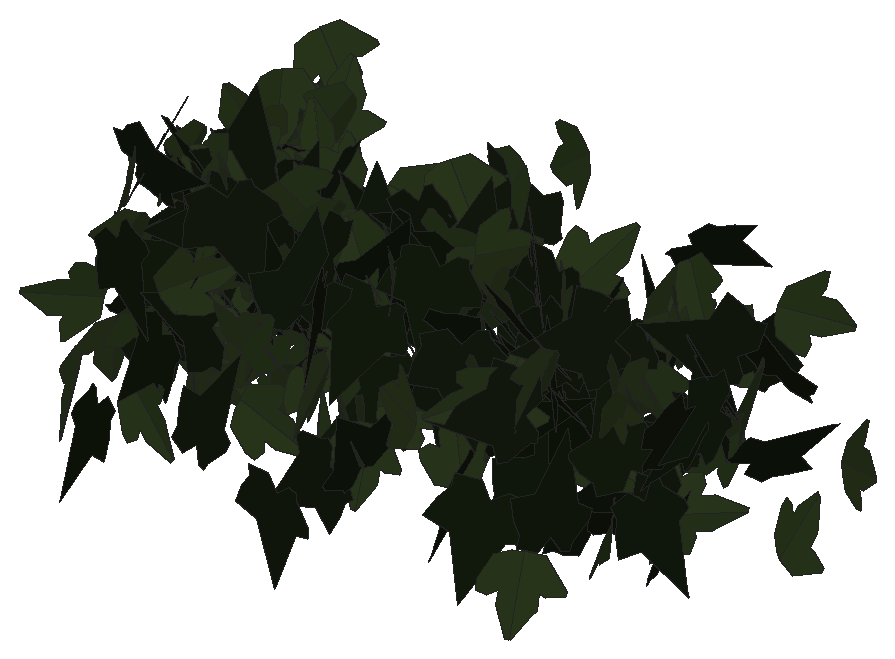
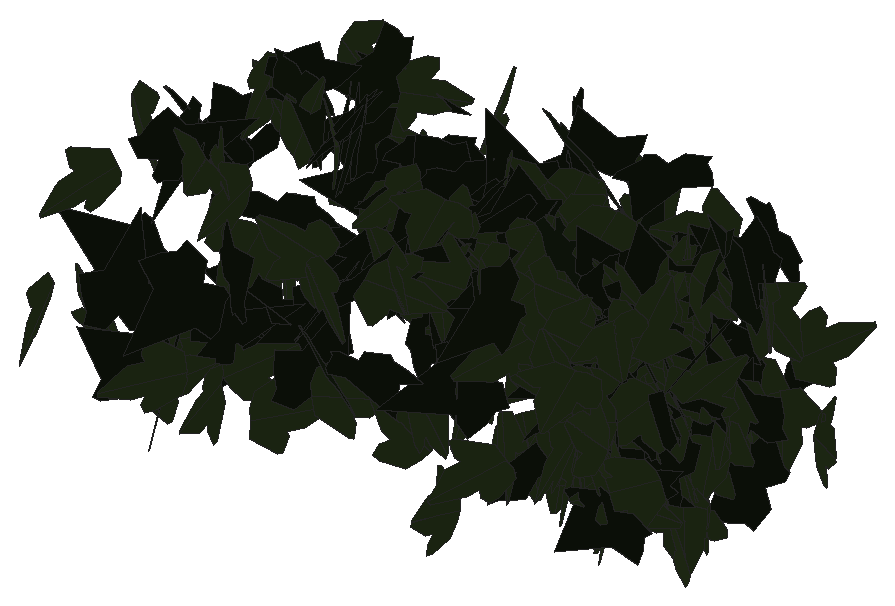
# SketchUp Ruby script. Lengths in inches.
U = 1.inch
M = Sketchup.active_model
def pt(a) = Geom::Point3d.new(a.map { |v| v * U })
def face(e, loops, mat)
  f = e.add_face(loops[0].map { |a| pt(a) })
  loops[1..].each { |l| e.add_face(l.map { |a| pt(a) }).erase! }
  f.material = f.back_material = mat if mat
  f
end
# faces: each face lists its corners as indices into pts; further lists are holes
def faces(e, pts, list, mat = nil) = list.each { |f| face(e, (f[0].is_a?(Array) ? f : [f]).map { |l| l.map { |i| pts[i] } }, mat) }
# xy, xz, yz: faces in a plane at the given z, y or x. An outline is a flat list of corners, or four numbers for a rectangle; further outlines are holes
def ring(l) = l.size == 4 ? [[l[0], l[1]], [l[2], l[1]], [l[2], l[3]], [l[0], l[3]]] : l.each_slice(2).to_a
def flat(e, list, mat, &to3) = list.each { |f| face(e, (f[0].is_a?(Array) ? f : [f]).map { |l| ring(l).map { |u, v| to3.(u, v) } }, mat) }
def xy(e, z, list, mat = nil) = flat(e, list, mat) { |x, y| [x, y, z] }
def xz(e, y, list, mat = nil) = flat(e, list, mat) { |x, z| [x, y, z] }
def yz(e, x, list, mat = nil) = flat(e, list, mat) { |y, z| [x, y, z] }
def lines(e, pts, list) = list.each { |a, b| e.add_line(pt(pts[a]), pt(pts[b])) }
# prism: a flat outline (further loops are holes) pulled along v
def prism(e, loops, v, mat = nil)
  f = face(e, loops, mat); d = Geom::Vector3d.new(v.map { |x| x * U })
  f.pushpull(f.normal.samedirection?(d) ? d.length : -d.length)
end
def box(e, o, s, mat = nil) = prism(e, [[o, [o[0] + s[0], o[1], o[2]], [o[0] + s[0], o[1] + s[1], o[2]], [o[0], o[1] + s[1], o[2]]]], [0, 0, s[2]], mat)
def at(x, y, z, deg = 0) = Geom::Transformation.translation(pt([x, y, z])) * Geom::Transformation.rotation(ORIGIN, Z_AXIS, deg.degrees)
def axes(o, x, y, z) = Geom::Transformation.new([*x, 0, *y, 0, *z, 0, *pt(o).to_a, 1])
def part(name) = M.definitions.add(name)
# library, detail: a bought-in or finely detailed component or shape, given as its bounding box
def library(name, o, s) = part(name).tap { |d| box(d.entities, o, s) }
def detail(e, o, s) = box(e.add_group.entities, o, s)
def put(e, d, t, mat = nil) = e.add_instance(d, t).tap { |i| i.material = mat if mat }
def group(e, t, mat = nil) = e.add_group.tap { |g| g.transformation = t; g.material = mat if mat }.entities
root = M.entities
M.materials.add("efeu1").color = [18, 25, 13]
M.materials.add("efeu2").color = [43, 57, 29]
c1 = part("ivyleaf_10")
p = [[0,0.5,-0.03],[-0.0625,2.02,-0.43],[-0.19,2.01,-0.46],[-0.54,1.05,-0.29],[-0.52,0.625,-0.18],[-0.83,0.76,-0.28],
  [-1.16,0.64,-0.33],[-1.15,0.33,-0.24],[-0.77,-0.39,0.02],[-0.3,-0.51,0.16],[0.04,-0.48,0.23],[-0.02,2.01,-0.4375],
  [-0.06,2.01,-0.43],[0.04,-0.49,0.23],[0.67,-0.49,0.14],[1.38,0.36,-0.2],[1.375,0.51,-0.24],[0.81,0.65,-0.19],
  [0.62,0.59,-0.15],[0.6,1.09,-0.28],[0.5,1.23,-0.31]]
faces(c1.entities,p,[[0,1,2,3,4,5,6,7,8,9,10],[11,12,0,13,14,15,16,17,18,19,20]],"efeu2")
c2 = part("ivyleaf_9")
p = [[1.54,2.16,1.25],[1.36,2.04,1.19],[-0.21,0.99,0.68],[-0.71,1.11,0.82],[-0.85,0.86,0.67],[-0.8,0.17,0.21],
  [-0.9,-0.01,0.1],[-0.67,-0.16,-0.02],[-0.08,-0.08,-0.05],[-0.03,-0.6,-0.4],[0.65,-0.88,-0.66],[0.83,-0.6,-0.49],
  [1.29,-0.42,-0.43],[1.8125,-0.07,-0.26],[1.21,0.44,0.15]]
faces(c2.entities,p,[[0,1,2,3,4,5,6,7,8,9,10,11,12,13,14]],"efeu1")
put(root,c1,axes([27.3,222.04,200.1875],[-0.07033,-0.07888,-0.4887],[-0.35362,-0.33742,0.10536],[-0.34641,0.36045,-0.00833]))
put(root,c1,axes([27.42,226.26,199.61],[-0.05716,-0.04905,0.49429],[-0.41545,-0.26801,-0.07464],[0.27227,-0.41924,-0.01011]))
put(root,c1,axes([27.09,223.93,200.35],[-0.19188,-0.43401,-0.15754],[0.07574,0.1387,-0.47437],[0.45546,-0.20591,0.01252]))
put(root,c1,axes([27.01,222.09,198.875],[0.1444,-0.2891,0.38154],[0.24601,-0.29705,-0.31819],[0.41064,0.27962,0.05645]))
put(root,c1,axes([27.26,223.02,201.81],[0.20835,-0.38864,-0.23569],[-0.08457,0.2216,-0.44016],[0.44659,0.22328,0.0266]))
put(root,c1,axes([27.37,224.38,198.55],[0.30131,-0.14229,0.37278],[-0.33716,0.15904,0.33322],[-0.2134,-0.45217,-0.0001]))
put(root,c1,axes([26.88,226.29,200.06],[-0.13135,-0.08792,-0.47436],[0.43987,0.18009,-0.15518],[0.19814,-0.45808,0.03004]))
put(root,c1,axes([27.35,224.56,200.51],[0.20097,0.30073,0.34521],[-0.18948,-0.28857,0.3617],[0.41678,-0.2762,-0.00202]))
put(root,c2,axes([26.8125,223.68,198.93],[0.37683,0.2117,-0.25137],[0.209,0.14077,0.43186],[0.25362,-0.43054,0.0176]))
put(root,c2,axes([27.04,223.67,199.8125],[-0.29008,0.08654,0.39795],[0.3557,-0.18409,0.29931],[0.19832,0.45675,0.04524]))
put(root,c1,axes([27.29,224.17,199.8],[-0.48393,-0.12229,-0.0293],[0.0293,0.00364,-0.49913],[0.12229,-0.4848,0.00365]))
put(root,c1,axes([27.22,223.58,199.55],[0.27582,-0.40414,0.10292],[-0.03477,0.10068,0.48852],[-0.41559,-0.27665,0.02743]))
put(root,c1,axes([27.33,222.58,199.48],[-0.13604,-0.47874,-0.04796],[0.0152,0.04554,-0.49769],[0.4809,-0.13687,0.00216]))
put(root,c1,axes([27.31,226.75,200.77],[0.15625,-0.33777,0.33391],[-0.12044,0.31184,0.37182],[-0.45943,-0.19663,0.01609]))
put(root,c1,axes([27.33,226.27,199.77],[0.19453,-0.35996,0.28737],[-0.11394,0.26465,0.40863],[-0.44629,-0.22447,0.02093]))
put(root,c1,axes([27.24,224.84,198.76],[0.4287,0.25582,0.02782],[0.02445,0.01332,-0.49922],[-0.25616,0.4294,-0.00109]))
put(root,c2,axes([27.09,226.68,199.72],[-0.08569,-0.16696,-0.46344],[0.35145,0.30889,-0.17627],[0.34516,-0.35597,0.06442]))
put(root,c1,axes([27.33,224.81,198.04],[0.34649,-0.36039,-0.00783],[0.00751,-0.00364,0.49993],[-0.3604,-0.34656,0.00289]))
put(root,c1,axes([27.48,222.72,201.07],[-0.01005,-0.42829,0.25781],[-0.01104,-0.25761,-0.42839],[0.49978,-0.0143,-0.00428]))
put(root,c2,axes([27.32,223.18,201.59],[-0.05837,0.46857,0.16444],[-0.01055,-0.1667,0.47127],[0.49647,0.05155,0.02935]))
put(root,c2,axes([27.31,224.41,201.21],[0.17979,-0.46655,-0.00314],[0.00549,0.00548,-0.49994],[0.46652,0.17974,0.0071]))
put(root,c1,axes([27.4,227.24,201.97],[0.33717,0.30468,0.20854],[0.15551,0.13894,-0.45444],[-0.33486,0.3713,-0.00107]))
put(root,c1,axes([27.8,225.18,201.6],[-0.35271,-0.26676,-0.23332],[-0.18786,-0.13839,0.44222],[-0.3005,0.39961,-0.0026]))
put(root,c1,axes([27.65,223.93,201.99],[0.09638,-0.37011,0.32207],[0.06944,-0.31463,-0.38234],[0.48568,0.11843,-0.00925]))
put(root,c1,axes([27.58,226.18,199.32],[-0.2742,0.35296,-0.22412],[0.12444,-0.18698,-0.44671],[-0.39916,-0.30076,0.01469]))
put(root,c2,axes([27.49,224.63,200.39],[-0.13298,-0.32593,-0.35509],[0.2092,0.29282,-0.34712],[0.43423,-0.24089,0.05849]))
put(root,c1,axes([27.51,224.125,199.21],[0.44672,0.06423,0.21521],[0.21356,0.02678,-0.4513],[-0.0695,0.49513,-0.00351]))
put(root,c2,axes([27.33,223.18,201.82],[0.15542,-0.10298,0.46394],[0.36711,-0.28395,-0.18601],[0.30178,0.39846,-0.01266]))
put(root,c1,axes([27.87,226.77,200.51],[-0.06593,0.13854,0.47588],[-0.21712,0.42348,-0.15337],[-0.44555,-0.22687,0.00432]))
put(root,c1,axes([27.74,225.82,202.03],[0.18161,0.45288,-0.10916],[-0.05059,-0.0973,-0.48782],[-0.4631,0.18824,0.01048]))
put(root,c2,axes([27.95,225.34,199.21],[-0.36742,-0.28648,0.18146],[-0.14429,-0.11005,-0.46591],[0.30689,-0.39474,-0.00181]))
put(root,c2,axes([28.14,224.19,200.18],[-0.10837,0.27977,0.39998],[-0.15325,0.3695,-0.29997],[-0.46343,-0.18761,0.00567]))
put(root,c1,axes([28.04,224.18,200.77],[-0.31541,-0.36909,0.11953],[-0.07312,-0.09473,-0.48547],[0.38101,-0.32372,0.00578]))
put(root,c1,axes([28.11,226.3125,200.95],[0.365,-0.21454,-0.26599],[-0.22414,0.14347,-0.42329],[0.25795,0.42824,0.00856]))
put(root,c2,axes([27.64,223.71,202.13],[0.36919,-0.31795,0.11227],[0.0844,-0.07405,-0.48723],[0.32646,0.37871,-0.001]))
put(root,c1,axes([27.97,222.53,199.82],[-0.31445,-0.3657,-0.13184],[0.0893,0.09709,-0.48229],[0.37834,-0.32686,0.00426]))
put(root,c1,axes([27.99,223.77,200.88],[-0.2236,-0.42823,-0.12894],[0.06716,0.11038,-0.48302],[0.44215,-0.23332,0.00816]))
put(root,c1,axes([28.1,226.24,200.41],[0.25308,-0.32535,-0.28301],[-0.14704,0.24338,-0.41127],[0.40537,0.2914,0.02751]))
put(root,c1,axes([28.07,226.17,201.02],[-0.08232,-0.43054,0.24053],[-0.03372,-0.23838,-0.43822],[0.49202,-0.08837,0.01021]))
put(root,c1,axes([27.77,224.6,200.2],[-0.38049,0.03511,-0.32248],[0.32135,-0.02703,-0.3821],[-0.04427,-0.49803,-0.002]))
put(root,c2,axes([27.84,224.12,200.0625],[-0.10863,0.36654,0.32225],[0.08099,-0.31202,0.38221],[0.48129,0.13524,0.00841]))
put(root,c2,axes([27.7,224.96,199.97],[-0.0605,0.09518,0.48711],[0.31232,-0.37408,0.11188],[0.38574,0.31781,-0.01419]))
put(root,c2,axes([27.6,224.61,199.21],[0.25899,-0.17627,0.38969],[0.31533,-0.22909,-0.31319],[0.28895,0.40798,-0.0075]))
put(root,c2,axes([28.18,222.92,199.16],[-0.26076,-0.38156,0.19084],[0.10878,0.1568,0.46215],[-0.41252,0.28253,0.00124]))
put(root,c1,axes([28.11,224.49,200.33],[-0.11788,-0.45417,0.17273],[-0.04,-0.16806,-0.46921],[0.48426,-0.12444,0.00329]))
put(root,c1,axes([28.13,226.2,200.08],[-0.24236,0.3906,0.1967],[-0.12578,0.15313,-0.45905],[-0.41886,-0.272,0.02404]))
put(root,c1,axes([27.86,225.04,200.46],[-0.3286,-0.11392,-0.35923],[0.34171,0.11091,-0.34775],[0.15891,-0.47405,0.00496]))
put(root,c1,axes([28.01,223.8,201.79],[0.46775,0.17662,-0.00405],[-0.00378,-0.00147,-0.49998],[-0.17663,0.46776,-0.00004]))
put(root,c1,axes([27.95,223.28,198.96],[-0.43919,-0.02888,0.23723],[0.23796,-0.00715,0.43968],[-0.022,0.49911,0.02003]))
put(root,c1,axes([27.98,226.37,200.25],[-0.43157,-0.15853,0.19652],[0.19576,0.03569,0.4587],[-0.15946,0.47286,0.03126]))
put(root,c2,axes([28.32,223.07,201.72],[0.16994,0.03273,-0.46909],[-0.4689,0.04939,-0.16642],[0.03545,0.49648,0.04748]))
put(root,c2,axes([28.01,224.75,201.625],[-0.28479,-0.24311,-0.33135],[0.28193,0.17774,-0.37272],[0.29901,-0.39913,0.03585]))
put(root,c1,axes([27.88,223.62,198.57],[0.04066,-0.02017,0.49794],[0.40181,-0.2942,-0.04473],[0.29479,0.40378,-0.00771]))
put(root,c2,axes([28.42,224.3125,200.18],[-0.14699,-0.08461,0.47036],[-0.33667,-0.33092,-0.16474],[0.33918,-0.36514,0.04031]))
put(root,c1,axes([28.12,226.51,201.32],[0.45982,0.14947,-0.12736],[0.12133,0.03874,0.48351],[0.1544,-0.47556,-0.00065]))
put(root,c2,axes([28.23,222.8,200.36],[-0.40763,0.12823,0.2596],[0.241,-0.09822,0.42693],[0.16049,0.47319,0.01827]))
put(root,c2,axes([28.13,222.57,200],[0.47425,0.1541,-0.03659],[-0.03475,-0.01144,-0.49866],[-0.15452,0.47552,-0.00014]))
put(root,c1,axes([28.21,224.03,201.8125],[0.0329,-0.13533,0.48021],[0.16604,-0.45085,-0.13843],[0.47048,0.16858,0.01528]))
put(root,c1,axes([28.46,224.31,199.58],[0.31494,-0.26592,-0.28302],[-0.22508,0.17195,-0.41203],[0.31646,0.38694,-0.0114]))
put(root,c1,axes([28.22,224.06,201.53],[-0.29463,0.18315,0.36007],[0.25057,-0.26673,0.34069],[0.31688,0.3812,0.06539]))
put(root,c2,axes([28.55,225.41,200.97],[-0.18925,0.45535,-0.08271],[0.02834,-0.07779,-0.4931],[-0.46193,-0.19132,0.00364]))
put(root,c1,axes([28.39,225.09,200.81],[-0.04526,-0.32082,-0.38082],[0.04278,0.37847,-0.32393],[0.49611,-0.0619,-0.00681]))
put(root,c1,axes([28.35,225.24,201.28],[0.27213,0.41055,-0.086],[-0.054,-0.06737,-0.49249],[-0.41597,0.27733,0.00767]))
put(root,c2,axes([28.45,224.03,201.53],[-0.34262,-0.18432,0.31407],[0.32012,0.05312,0.3804],[-0.1736,0.46174,0.08161]))
put(root,c1,axes([28.48,226.17,201.83],[-0.01565,-0.29161,0.40586],[0.02433,-0.40602,-0.29079],[0.49916,0.01065,0.0269]))
put(root,c2,axes([28.37,220.87,199.25],[-0.03083,0.03049,-0.49812],[0.35617,-0.34823,-0.04336],[-0.34956,-0.3575,-0.00025]))
put(root,c2,axes([28.22,221.5625,201.58],[-0.14559,-0.08339,-0.47101],[0.46186,0.10358,-0.1611],[0.12444,-0.48199,0.04686]))
put(root,c2,axes([28.73,223.57,201.125],[-0.17445,-0.11164,0.45509],[-0.35856,-0.28083,-0.20634],[0.30167,-0.39834,0.01792]))
put(root,c1,axes([28.32,224.43,200.8],[-0.28325,-0.17453,-0.37324],[0.33935,0.15807,-0.33145],[0.23369,-0.44108,0.02891]))
put(root,c1,axes([28.3,223.55,198.8],[-0.36215,-0.01763,-0.34429],[0.34372,0.01993,-0.36258],[0.0265,-0.49929,-0.00232]))
put(root,c1,axes([28.9,224.34,200.44],[-0.24608,0.06685,-0.43009],[-0.4187,0.0986,0.25489],[0.11889,0.4856,0.00745]))
put(root,c1,axes([28.36,223.27,201.67],[0.2992,-0.2124,0.33966],[0.28043,-0.19168,-0.3669],[0.28607,0.41005,0.00443]))
put(root,c2,axes([28.27,225.39,201.18],[0.44539,0.06097,0.21887],[0.2132,0.05437,-0.44899],[-0.07855,0.49328,0.02243]))
put(root,c1,axes([28.25,221.95,198.91],[0.27941,-0.02178,0.41407],[0.41449,0.00109,-0.27964],[0.01128,0.49952,0.01867]))
put(root,c2,axes([28.5,222.15,199.89],[0.09441,-0.1581,-0.46486],[0.31564,-0.34306,0.18078],[-0.37611,-0.32759,0.03503]))
put(root,c1,axes([28.86,225.71,200.82],[0.09567,0.13923,0.4706],[-0.24015,-0.40485,0.16859],[0.42799,-0.25828,-0.01059]))
put(root,c1,axes([28.6875,225.47,201.23],[0.12935,0.48062,-0.04764],[0.01192,0.04613,0.49772],[0.48283,-0.1299,0.00048]))
put(root,c2,axes([28.36,223.88,200.72],[-0.03737,-0.02611,-0.49792],[0.35753,0.34662,-0.04501],[0.34753,-0.3594,-0.00724]))
put(root,c1,axes([28.92,224.41,198.11],[0.41233,-0.03605,0.28051],[-0.27994,0.0185,0.41387],[-0.04021,-0.49836,-0.00493]))
put(root,c1,axes([28.42,224.54,201.65],[0.07943,-0.06321,-0.48959],[0.42344,-0.24617,0.10048],[-0.25375,-0.43059,0.01442]))
put(root,c1,axes([29.11,223.48,199.66],[0.03893,0.02272,0.49796],[-0.33941,-0.3646,0.04317],[0.36508,-0.34139,-0.01297]))
put(root,c1,axes([28.92,223.35,201.35],[-0.06999,-0.31843,0.37909],[-0.03004,-0.37942,-0.32425],[0.49417,-0.06816,0.03398]))
put(root,c2,axes([29.09,223.43,199.52],[0.02913,-0.03667,0.4978],[-0.16512,0.46987,0.04428],[-0.47105,-0.16698,0.01526]))
put(root,c1,axes([28.91,225.38,199.21],[-0.18491,0.4051,0.22738],[0.07973,-0.21343,0.44507],[0.45766,0.20086,0.01434]))
put(root,c1,axes([28.96,224.65,198.25],[-0.1013,-0.35365,-0.33863],[-0.05429,-0.33555,0.36668],[-0.48661,0.11106,0.02958]))
put(root,c1,axes([28.83,227.22,200.07],[0.14836,0.2147,0.42649],[0.25695,0.34052,-0.26081],[-0.40245,0.29656,-0.00929]))
put(root,c2,axes([29.2,222,200.91],[-0.15315,0.22305,-0.42047],[-0.23616,0.34788,0.27056],[0.41325,0.28147,-0.0012]))
put(root,c1,axes([29.1875,223.45,199.12],[-0.26513,-0.37775,-0.19238],[-0.10779,-0.15937,0.4615],[-0.40998,0.28619,0.00307]))
put(root,c2,axes([29.12,223.5,199.9],[0.19539,0.33662,0.31386],[0.14635,0.27784,-0.38909],[-0.43635,0.24391,0.01005]))
put(root,c1,axes([29.22,223.46,200.8125],[-0.18698,-0.45544,-0.08725],[0.03539,0.07979,-0.49232],[0.46237,-0.19028,0.0024]))
put(root,c1,axes([29.21,225.14,200.22],[0.49264,0.05738,0.06336],[-0.06303,-0.0065,0.49597],[0.05774,-0.49665,0.00082]))
put(root,c2,axes([29.05,225.33,200.2],[0.10933,-0.48399,-0.06166],[-0.01262,0.06037,-0.49618],[0.48774,0.11005,0.00098]))
put(root,c2,axes([29.26,224.57,201.49],[0.00894,-0.17154,-0.46957],[0.16861,-0.44109,0.16435],[-0.47063,-0.16129,0.04996]))
put(root,c2,axes([29.33,222.21,200.33],[0.08912,-0.47773,-0.1176],[0.0559,-0.1089,0.48478],[-0.48881,-0.09956,0.034]))
put(root,c2,axes([29.41,224.26,200.15],[0.16657,0.44948,-0.14219],[-0.05531,-0.13114,-0.47932],[-0.46818,0.17541,0.00604]))
put(root,c1,axes([29.69,224.91,201.59],[0.0575,0.07518,0.49096],[-0.48955,-0.07489,0.0688],[0.08388,-0.48861,0.065]))
put(root,c2,axes([29.25,222.06,198.54],[-0.29066,0.30266,0.27188],[0.18142,-0.20266,0.41955],[0.36415,0.34253,0.00799]))
put(root,c1,axes([29.22,221.64,201.18],[-0.04187,-0.16171,0.47127],[0.1854,0.43391,0.16536],[-0.46246,0.1886,0.02362]))
put(root,c1,axes([29.23,224.52,200.54],[0.18524,-0.20504,0.41671],[0.27222,-0.31554,-0.27627],[0.37627,0.32923,-0.00527]))
put(root,c1,axes([29.55,224.63,199.08],[-0.35669,-0.34272,-0.07294],[0.05259,0.05054,-0.49465],[0.34642,-0.36054,-0.00001]))
put(root,c2,axes([29.49,223.72,201.15],[-0.21291,-0.19875,0.40641],[0.35036,0.21173,0.28709],[-0.28621,0.40703,0.04911]))
put(root,c2,axes([29.18,223.58,200.07],[0.41625,-0.09119,0.26157],[0.25784,-0.04502,-0.42602],[0.10125,0.48955,0.00954]))
put(root,c1,axes([29.55,224.23,199.8],[-0.21459,-0.29867,-0.33875],[0.18181,0.28617,-0.36749],[0.41339,-0.2809,-0.01422]))
put(root,c2,axes([29.45,223.1,201.33],[-0.23676,-0.03365,-0.43911],[0.43,0.09002,-0.23874],[0.09513,-0.49068,-0.01369]))
put(root,c2,axes([29.35,223.9,200.07],[0.17699,-0.31741,0.3434],[0.19537,-0.2834,-0.36265],[0.42486,0.26255,0.0237]))
put(root,c1,axes([29.63,223.6,202.05],[-0.27956,-0.30592,-0.27975],[0.19352,0.20209,-0.41438],[0.3666,-0.33997,0.00541]))
put(root,c1,axes([29.39,223.12,198.58],[0.17798,0.06918,0.4621],[0.42967,0.17006,-0.19095],[-0.18359,0.46508,0.00109]))
put(root,c2,axes([29.86,225.43,198.81],[0.05011,-0.32766,-0.37434],[0.04496,-0.37171,0.33138],[-0.49545,-0.06687,-0.00778]))
put(root,c2,axes([30.02,224.23,202.07],[-0.32799,0.37554,-0.03725],[0.02419,-0.02833,-0.49861],[-0.37661,-0.32888,0.00041]))
put(root,c2,axes([29.55,224.29,200.88],[0.27459,-0.41294,0.06391],[0.03372,-0.05433,-0.49589],[0.41649,0.27664,-0.00199]))
put(root,c2,axes([29.66,222.24,202.44],[-0.07769,-0.39164,-0.30096],[0.11481,0.282,-0.3966],[0.4804,-0.13073,0.04612]))
put(root,c1,axes([29.97,225.46,199.49],[0.12621,-0.43088,-0.22003],[-0.06264,0.21092,-0.44898],[0.47974,0.1409,-0.00074]))
put(root,c1,axes([30.0625,223.95,200.3125],[-0.4746,-0.08441,0.13279],[-0.1308,-0.02286,-0.48205],[0.08745,-0.49229,-0.00038]))
put(root,c2,axes([29.57,223.8,200.3],[0.21447,-0.03765,0.45009],[0.45124,-0.00363,-0.21533],[0.01949,0.49857,0.03242]))
put(root,c1,axes([29.88,224.25,200.12],[0.07301,-0.15621,0.46933],[0.22723,-0.4108,-0.17208],[0.43936,0.23842,0.01101]))
put(root,c1,axes([30.32,224.59,198.97],[-0.29979,-0.39002,0.0895],[-0.05481,-0.07076,-0.49192],[0.39638,-0.30476,-0.00033]))
put(root,c1,axes([30.25,222.53,200.73],[0.10057,-0.41602,0.25848],[0.06037,-0.25134,-0.428],[0.48605,0.11729,-0.00032]))
put(root,c1,axes([30.32,223.6,201.87],[0.01422,-0.4286,0.2571],[0.00256,-0.25714,-0.4288],[0.49979,0.01351,-0.00512]))
put(root,c2,axes([30.18,222.19,200.52],[0.41154,-0.28078,-0.04237],[0.03891,-0.01814,0.49815],[-0.28128,-0.41332,0.00693]))
put(root,c1,axes([30.4375,224.16,199.71],[0.33164,0.25162,-0.27695],[-0.22186,-0.16579,-0.41629],[-0.30132,0.399,0.00168]))
put(root,c1,axes([30.36,223.22,201.32],[0.19186,-0.43779,0.14671],[0.05869,-0.13446,-0.47799],[0.45798,0.20064,-0.0002]))
put(root,c2,axes([30.12,223.47,200.39],[0.11733,0.02306,0.48549],[0.44655,0.19208,-0.11704],[-0.1919,0.46106,0.02447]))
put(root,c2,axes([30.19,225.15,201.35],[0.49151,-0.09177,0.00032],[0.00071,0.00207,-0.5],[0.09177,0.4915,0.00217]))
put(root,c1,axes([30.26,224.73,201.22],[-0.39662,-0.00213,-0.30445],[0.30434,0.01079,-0.39656],[0.00826,-0.49988,-0.00726]))
put(root,c1,axes([30.22,224.89,200.52],[-0.20374,-0.14855,-0.43177],[0.37257,0.21925,-0.25124],[0.26397,-0.4241,0.02135]))
put(root,c1,axes([30.56,226.03,198.21],[0.08107,-0.16201,0.46603],[-0.16766,0.43513,0.18043],[-0.46402,-0.18552,0.01623]))
put(root,c1,axes([30.4375,224.02,201.55],[-0.40859,0.04328,-0.28493],[0.28199,-0.04199,-0.41075],[-0.05948,-0.49635,0.0099]))
put(root,c2,axes([30.82,224.45,201.14],[0.05197,-0.47748,0.13897],[-0.00691,0.13902,0.48023],[-0.49724,-0.05184,0.00785]))
put(root,c1,axes([30.84,222.8125,198.4],[0.36905,-0.21407,0.26073],[-0.2205,0.13939,0.42656],[-0.25531,-0.42982,0.00848]))
put(root,c2,axes([30.38,223.89,200.23],[0.05905,-0.01164,0.49636],[0.47964,-0.12782,-0.06006],[0.12829,0.48325,-0.00393]))
put(root,c1,axes([30.82,222.82,201.89],[-0.2553,-0.34219,-0.26025],[0.15333,0.21029,-0.42693],[0.40164,-0.2978,-0.00244]))
put(root,c1,axes([30.68,221.3,200.93],[-0.39666,-0.0312,0.30279],[0.30303,0.00653,0.39765],[-0.02877,0.49898,0.01373]))
put(root,c2,axes([30.82,223.82,201.08],[-0.02531,0.2357,-0.44024],[-0.10625,0.42816,0.23534],[0.48792,0.10547,0.02842]))
put(root,c1,axes([30.92,224.62,201.34],[0.12017,-0.45148,0.17811],[0.0542,-0.16985,-0.46713],[0.48231,0.13158,0.00812]))
put(root,c2,axes([30.74,225.14,199.92],[0.08148,0.10688,-0.4816],[0.12282,0.46836,0.12472],[0.47778,-0.13863,0.05007]))
put(root,c1,axes([31.08,224.8,199.55],[-0.00193,-0.32309,-0.38159],[-0.01783,0.38139,-0.32284],[0.49968,0.01236,-0.01299]))
put(root,c2,axes([30.89,224.48,200.64],[-0.03082,-0.21096,-0.45227],[0.14752,0.42903,-0.21018],[0.47675,-0.1464,0.0358]))
put(root,c2,axes([31.2,223.78,200.88],[0.38863,0.10125,-0.29785],[-0.29142,-0.06242,-0.40147],[-0.11849,0.48564,0.0105]))
put(root,c2,axes([31.29,223.49,201.44],[-0.37384,-0.20463,0.26147],[0.23409,0.1168,0.4261],[-0.23546,0.44101,0.00848]))
put(root,c2,axes([31.57,222.125,202.25],[-0.35121,0.32091,0.15385],[-0.12549,0.0906,-0.47544],[-0.33302,-0.37257,0.0169]))
put(root,c2,axes([31.57,223.94,201.86],[0.07808,0.17405,-0.46218],[-0.26004,-0.38331,-0.18828],[-0.41986,0.26978,0.03066]))
put(root,c1,axes([31.07,223.64,201.16],[0.13041,0.10542,-0.47104],[0.36027,0.30348,0.16766],[0.32125,-0.38313,0.0032]))
put(root,c1,axes([31.07,223.2,202],[0.40262,0.03755,0.29409],[0.29328,0.02221,-0.40434],[-0.04343,0.49809,-0.00414]))
put(root,c2,axes([31.4,221.68,201.57],[-0.35632,-0.15819,0.31307],[0.28334,0.13325,0.38982],[-0.20676,0.45521,-0.00532]))
put(root,c2,axes([31.71,223.66,199.43],[-0.41119,-0.18063,0.21976],[-0.20261,-0.08517,-0.4491],[0.19968,-0.45839,-0.00315]))
put(root,c1,axes([31.71,226.07,201.51],[0.19023,0.16397,-0.43235],[-0.37054,-0.22561,-0.24859],[-0.27661,0.41498,0.03568]))
put(root,c1,axes([31.71,224.03,200.08],[0.19214,-0.11401,0.44731],[-0.37155,0.24932,0.22314],[-0.27392,-0.41814,0.01108]))
put(root,c2,axes([31.16,223.78,200.72],[0.17997,-0.28717,0.36762],[0.20486,-0.30535,-0.33881],[0.4191,0.27258,0.00775]))
put(root,c1,axes([31.36,223.05,199.11],[0.06176,-0.06213,0.49227],[0.37113,-0.32346,-0.08739],[0.32931,0.37619,0.00616]))
put(root,c2,axes([31.42,224.32,202.08],[0.17792,-0.44155,-0.15289],[-0.0402,0.14852,-0.47574],[0.46554,0.18158,0.01735]))
put(root,c2,axes([31.98,225.02,201.03],[-0.29388,-0.05779,0.40036],[-0.38811,-0.09922,-0.29921],[0.11403,-0.48664,0.01346]))
put(root,c1,axes([31.84,225.92,202.02],[0.37888,-0.2186,-0.24221],[-0.19774,0.14139,-0.43693],[0.25952,0.42688,0.02068]))
put(root,c2,axes([31.5,223.09,201.53],[0.34713,0.341,0.11497],[-0.08389,-0.07867,0.48659],[0.34995,-0.35711,0.00259]))
put(root,c1,axes([31.48,224.9,201.08],[-0.10524,-0.17053,0.45809],[0.28243,0.36123,0.19936],[-0.39894,0.30072,0.0203]))
put(root,c1,axes([31.52,224.98,202.28],[0.37716,0.24674,0.2165],[0.18205,0.11719,-0.45069],[-0.27315,0.41879,-0.00144]))
put(root,c1,axes([31.77,225.05,199.1],[0.08758,-0.45219,0.19455],[0.05546,-0.18729,-0.46027],[0.48914,0.1022,0.01735]))
put(root,c2,axes([31.75,221.84,199.07],[0.16152,-0.28711,-0.37614],[0.17616,-0.3324,0.32937],[-0.43918,-0.23891,-0.00622]))
put(root,c1,axes([32.06,227.0625,201.91],[0.26826,-0.18273,-0.38032],[-0.28965,0.24797,-0.32344],[0.30682,0.39386,0.02719]))
put(root,c2,axes([31.9,226.29,200.27],[-0.40029,-0.26564,-0.13856],[0.11509,0.07716,-0.48042],[0.27662,-0.41651,-0.00063]))
put(root,c1,axes([31.81,222.61,199.1875],[0.49985,0.00997,0.00693],[0.0069,0.00164,-0.49995],[-0.00999,0.4999,0.0015]))
put(root,c2,axes([32.14,225.9375,201.125],[-0.3087,-0.37614,0.11497],[0.07338,0.08851,0.4866],[-0.38642,0.3173,0.00056]))
put(root,c2,axes([31.79,221.65,202.04],[-0.12116,0.06177,-0.48115],[0.42572,-0.22422,-0.13598],[-0.23256,-0.44262,0.00173]))
put(root,c1,axes([31.83,221.54,200.67],[0.08993,-0.18733,0.45478],[0.22779,-0.39388,-0.20729],[0.43592,0.24447,0.0145]))
put(root,c1,axes([31.77,223.26,201.64],[-0.14368,0.11394,0.46516],[0.36627,-0.28674,0.18338],[0.30855,0.39344,-0.00107]))
put(root,c2,axes([32.03,222.51,201.42],[-0.31025,-0.3921,0.0016],[-0.00081,-0.00139,-0.5],[0.3921,-0.31026,0.00023]))
put(root,c1,axes([32.19,221.89,199.52],[-0.3349,0.3111,-0.20264],[-0.14976,0.13652,0.45709],[0.33973,0.36685,0.00174]))
put(root,c1,axes([32.1,224.28,200.81],[-0.07085,-0.49374,-0.03458],[0.00639,0.03402,-0.4988],[0.49491,-0.07113,0.00149]))
put(root,c1,axes([32,224.9,198.38],[-0.10136,-0.39248,0.29272],[0.05927,0.28689,0.40519],[-0.48602,0.11684,-0.01164]))
put(root,c1,axes([31.77,224.31,201.51],[-0.1886,-0.0817,0.4558],[0.42954,0.15299,0.20516],[-0.17299,0.46895,0.01248]))
put(root,c2,axes([32.27,223.67,200.17],[-0.13988,0.34374,-0.33507],[0.13171,-0.30813,-0.37109],[-0.46161,-0.19208,-0.00435]))
put(root,c2,axes([32.18,224.45,201.14],[-0.42661,0.00615,0.2607],[0.26074,0.00301,0.42662],[0.00368,0.49995,-0.00578]))
put(root,c1,axes([31.92,223.17,199.49],[0.0335,-0.00397,0.49886],[0.32508,0.37943,-0.01881],[-0.37842,0.3256,0.028]))
put(root,c2,axes([32.32,221.85,199.33],[0.156,0.20756,0.4273],[-0.24103,-0.35297,0.25945],[0.40935,-0.28693,-0.01007]))
put(root,c1,axes([32.35,223.53,200.61],[0.495,-0.06527,0.02669],[-0.02472,0.0166,0.49911],[-0.06604,-0.49544,0.0132]))
put(root,c2,axes([32.49,223.4,201.83],[-0.25499,-0.4124,-0.12209],[0.07091,0.09969,-0.4848],[0.42421,-0.26455,0.00765]))
put(root,c2,axes([32.42,219.85,199.73],[0.05301,-0.47296,0.15328],[0.0279,-0.15108,-0.47581],[0.4964,0.059,0.01037]))
put(root,c2,axes([32.41,224.53,200.83],[0.4081,-0.27236,0.09631],[0.0813,-0.05167,-0.49063],[0.27721,0.41612,0.00211]))
put(root,c1,axes([32.7,224.23,201.85],[-0.00393,-0.12589,-0.48388],[0.20262,0.44198,-0.11664],[0.45709,-0.197,0.04754]))
put(root,c1,axes([32.89,224.04,201.19],[-0.00818,-0.33467,-0.37139],[0.00432,0.37138,-0.33476],[0.49991,-0.00868,-0.00318]))
put(root,c2,axes([32.85,223.34,200.18],[-0.37566,-0.14343,-0.29716],[0.27302,0.11775,-0.40199],[0.18529,-0.46429,-0.01015]))
put(root,c1,axes([33.36,225.15,198.74],[-0.0381,-0.00805,-0.49848],[-0.49654,-0.04418,0.03867],[-0.04467,0.49798,-0.00463]))
put(root,c2,axes([33.4,225.26,199.29],[-0.3853,0.18456,-0.25977],[-0.24756,0.08326,0.42636],[0.20063,0.45717,0.02722]))
put(root,c1,axes([33.28,222.85,199.2],[0.13836,0.47749,-0.05348],[-0.00103,0.05595,0.49686],[0.48048,-0.13738,0.01646]))
put(root,c2,axes([33.29,223.13,199.09],[-0.18884,0.17186,-0.42989],[0.30141,-0.30677,-0.25504],[-0.35141,-0.35547,0.01226]))
put(root,c2,axes([32.97,222.88,201.24],[0.41409,0.02693,0.27894],[0.27764,0.02809,-0.41488],[-0.03801,0.49848,0.00832]))
put(root,c1,axes([33.38,225.54,201.17],[0.27187,0.16915,-0.38402],[0.32023,0.21207,0.32012],[0.27118,-0.42002,0.00698]))
put(root,c1,axes([33.68,227.32,199.6],[0.00553,-0.07104,-0.4949],[0.02323,0.49443,-0.07071],[0.49943,-0.02221,0.00877]))
put(root,c2,axes([33.72,225.11,198.63],[0.21374,0.1601,0.42271],[-0.34306,-0.24701,0.26701],[0.29432,-0.40417,0.00426]))
put(root,c2,axes([33.38,223.77,200.67],[0.17237,-0.31636,0.34671],[0.1873,-0.2923,-0.35983],[0.43036,0.25393,0.01774]))
put(root,c2,axes([33.88,224.03,200.28],[-0.01921,-0.37571,-0.32935],[-0.01648,-0.32894,0.3762],[-0.49936,0.02531,0.00026]))
put(root,c2,axes([33.5,224.98,200.18],[0.22045,-0.44601,-0.04971],[-0.01825,0.04643,-0.4975],[0.4484,0.22117,0.0042]))
put(root,c1,axes([33.77,221.06,200.95],[-0.21215,0.34681,0.29106],[0.13102,-0.26064,0.40608],[0.43339,0.24857,0.01971]))
put(root,c2,axes([33.6875,222.43,201.41],[-0.19736,-0.37641,-0.26337],[0.12141,0.23372,-0.42501],[0.44307,-0.23171,-0.00085]))
put(root,c1,axes([34.13,225.6,198.34],[0.01737,0.0052,-0.49967],[-0.36131,-0.34525,-0.01615],[-0.34519,0.36163,-0.00824]))
put(root,c1,axes([33.61,225.22,200.54],[-0.16253,0.04407,0.47079],[0.45757,-0.11085,0.16834],[0.11921,0.48556,-0.0043]))
put(root,c2,axes([34.21,223.57,201.71],[0.07763,-0.24483,0.42899],[-0.04567,0.42883,0.25301],[-0.49182,-0.07847,0.04422]))
put(root,c2,axes([33.83,224.0625,202.03],[0.15632,-0.07507,-0.46897],[0.42143,-0.20574,0.1734],[-0.21901,-0.44948,-0.00105]))
put(root,c1,axes([34.17,223.125,200.52],[0.02704,-0.38693,0.31552],[0.03891,-0.31338,-0.38766],[0.49775,0.04552,0.01316]))
put(root,c2,axes([34.08,227.18,201.14],[0.34825,0.31332,0.17479],[0.127,0.12016,-0.46844],[-0.33555,0.37066,0.00411]))
put(root,c2,axes([34.34,222.94,199.14],[-0.41318,0.27687,0.05121],[0.03973,-0.03271,0.49734],[0.27875,0.41506,0.00503]))
put(root,c2,axes([34.28,222.26,199.2],[-0.28755,-0.40327,-0.0685],[0.04157,0.05449,-0.49528],[0.40692,-0.29053,0.00219]))
put(root,c1,axes([33.96,222.4,200.77],[-0.13036,-0.0005,0.48271],[0.47994,-0.05361,0.12956],[0.05163,0.49712,0.01445]))
put(root,c2,axes([34.19,223.94,202.12],[0.01378,-0.47215,0.16397],[0.01548,-0.16355,-0.47224],[0.49957,0.01809,0.01011]))
put(root,c1,axes([34.55,223.57,201.59],[0.21536,-0.17211,0.41713],[-0.33524,0.24836,0.27555],[-0.30205,-0.39837,-0.00842]))
put(root,c2,axes([34.71,225.68,200.29],[0.04343,-0.09945,0.48808],[-0.17208,0.45677,0.10839],[-0.46744,-0.17739,0.00545]))
put(root,c2,axes([34.39,222.34,200.35],[0.13481,0.06483,0.4771],[0.43706,0.19138,-0.1495],[-0.202,0.45735,-0.00507]))
put(root,c1,axes([34.93,221.56,201.5],[0.12988,0.09289,-0.47382],[-0.38449,-0.27689,-0.15968],[-0.29206,0.40583,-0.0005]))
put(root,c2,axes([34.71,224.61,201.09],[-0.34646,-0.30395,-0.19385],[0.14226,0.13176,-0.46087],[0.33125,-0.3745,-0.00482]))
put(root,c1,axes([34.55,227.31,199.58],[0.00902,0.04176,0.49817],[0.17868,0.46507,-0.04222],[-0.4669,0.17879,-0.00653]))
put(root,c2,axes([34.39,222.47,202.31],[0.3705,-0.25411,0.21945],[0.18222,-0.12231,-0.44926],[0.282,0.41288,0.00197]))
put(root,c1,axes([34.64,222.09,200.89],[0.48,0.06382,-0.12462],[0.12297,0.02061,0.4842],[0.06694,-0.49548,0.00409]))
put(root,c2,axes([34.79,223.34,201.57],[-0.08928,-0.38872,0.30154],[-0.07389,-0.2924,-0.3988],[0.48638,-0.11578,-0.00524]))
put(root,c1,axes([35.11,225.01,198.4],[0.22009,0.20439,0.39973],[-0.30503,-0.25857,0.30016],[0.32942,-0.37599,0.01087]))
put(root,c2,axes([34.8125,223.42,198.64],[-0.01496,0.24988,-0.43282],[-0.09752,0.42323,0.24772],[0.49017,0.09183,0.03607]))
put(root,c2,axes([34.54,222.74,201.31],[0.28862,-0.26165,0.31342],[0.24781,-0.19278,-0.38914],[0.32448,0.37997,0.0184]))
put(root,c2,axes([35.19,225.53,199.13],[-0.15905,-0.12883,0.45619],[-0.36187,-0.27781,-0.20462],[0.30619,-0.39525,-0.00487]))
put(root,c2,axes([34.78,223.07,201.61],[0.04139,-0.00102,-0.49828],[0.46524,-0.17897,0.03901],[-0.17843,-0.46687,-0.01386]))
put(root,c1,axes([35.11,225.03,201.3],[-0.00986,0.09171,0.49142],[-0.15101,0.46801,-0.09037],[-0.47655,-0.1502,0.01846]))
put(root,c2,axes([35.14,226.41,199.4],[0.2251,-0.11228,-0.43212],[-0.38286,0.20041,-0.25151],[0.22968,0.44411,0.00425]))
put(root,c2,axes([35.14,222.6,198.91],[-0.19609,-0.24428,0.38972],[0.25964,0.29091,0.31298],[-0.37965,0.32512,0.01276]))
put(root,c1,axes([35.05,224.82,200.4375],[-0.46453,-0.05351,-0.17706],[0.17575,0.02155,-0.4676],[0.05767,-0.49666,-0.00121]))
put(root,c1,axes([35.08,223.75,201.62],[-0.02665,-0.23718,-0.43936],[-0.00876,-0.43969,0.23789],[-0.49921,0.02038,0.01928]))
put(root,c2,axes([35.54,221.45,201.44],[-0.3843,0.03649,0.31778],[-0.3163,0.03066,-0.38603],[-0.04766,-0.49772,-0.00048]))
put(root,c2,axes([35.05,227.31,199.47],[-0.10713,-0.0774,0.48222],[0.39634,0.27469,0.13214],[-0.28538,0.41055,0.0025]))
put(root,c2,axes([35.5,223.11,202.18],[-0.16108,0.45138,0.1425],[-0.05237,0.13261,-0.47924],[-0.47044,-0.16932,0.00456]))
put(root,c1,axes([35.34,226.42,198.8125],[-0.03065,0.07386,-0.49356],[-0.15983,-0.4699,-0.06039],[-0.47278,0.15407,0.05241]))
put(root,c2,axes([35.7,224.59,199.34],[-0.30937,-0.07472,-0.38563],[-0.37529,-0.08869,0.31826],[-0.11596,0.48637,-0.0012]))
put(root,c2,axes([35.63,223.74,199.65],[-0.39796,-0.27158,0.13368],[0.11613,0.06693,0.4817],[-0.27953,0.41445,0.00981]))
put(root,c2,axes([35.83,223.08,202.02],[-0.26733,-0.13359,0.40086],[-0.36062,-0.17508,-0.29884],[0.2202,-0.44889,-0.00274]))
put(root,c2,axes([35.45,223.6875,198.84],[0.37814,0.32443,0.04189],[0.02616,0.03383,-0.49817],[-0.32608,0.37895,0.00861]))
put(root,c1,axes([35.57,221.89,202.04],[0.06749,-0.42405,0.25618],[0.06341,-0.24903,-0.42891],[0.49135,0.09039,0.02017]))
put(root,c1,axes([35.39,225.43,201.85],[0.38766,-0.02219,0.31501],[0.31314,-0.03749,-0.38799],[0.04084,0.4981,-0.01517]))
put(root,c1,axes([35.39,225.02,201.42],[0.0567,-0.01999,0.49637],[0.43495,-0.23937,-0.05932],[0.24001,0.43852,-0.00976]))
put(root,c1,axes([35.9375,222.89,199.11],[0.12778,-0.39486,-0.27885],[-0.08738,0.26481,-0.41502],[0.47543,0.15479,-0.00134]))
put(root,c1,axes([35.9,220.96,199.29],[0.41668,0.27166,-0.0508],[-0.04273,-0.02747,-0.49741],[-0.27305,0.41886,0.00032]))
put(root,c2,axes([35.89,226.72,199.9],[0.45165,-0.17439,0.12489],[-0.11632,0.04547,0.48415],[-0.18022,-0.46639,0.0005]))
put(root,c1,axes([35.79,224.57,198.6],[-0.02193,-0.04143,-0.4978],[0.41862,0.27034,-0.04095],[0.27254,-0.41857,0.02283]))
put(root,c2,axes([36.25,223.57,198.48],[0.01472,0.14962,0.47686],[0.08637,0.46913,-0.14986],[-0.49226,0.08678,-0.01203]))
put(root,c2,axes([36.6,224.86,201.28],[-0.08608,-0.02382,0.49196],[-0.46997,-0.14545,-0.08927],[0.14736,-0.47778,0.00265]))
put(root,c1,axes([36.45,222.55,201.64],[-0.06049,-0.32778,-0.37269],[0.07184,0.36571,-0.33331],[0.4911,-0.09388,0.00285]))
put(root,c1,axes([36.15,222.79,201.35],[-0.111,0.03374,0.48636],[0.466,-0.13925,0.11601],[0.14328,0.47903,-0.00053]))
put(root,c2,axes([36.5625,224.18,201.45],[0.41051,-0.08955,-0.27104],[-0.25661,0.09218,-0.41911],[0.12503,0.4832,0.02972]))
put(root,c2,axes([36.77,222.93,200.72],[0.10105,0.17266,0.45823],[0.2585,0.37857,-0.19965],[-0.41589,0.27726,-0.01276]))
put(root,c2,axes([37.07,223.48,200.97],[-0.43467,0.22166,-0.10922],[0.09415,-0.05577,-0.48788],[-0.22846,-0.4447,0.00675]))
put(root,c1,axes([36.75,226.06,201.49],[0.04882,0.2,0.45565],[0.106,0.44315,-0.20587],[-0.48619,0.1167,0.00087]))
put(root,c2,axes([36.82,225.08,199.54],[0.28236,0.38477,-0.14907],[0.08691,0.12113,0.47726],[0.40339,-0.29543,0.00152]))
put(root,c2,axes([37.44,223.44,201.27],[-0.4765,0.15142,0.00433],[-0.00477,-0.00072,-0.49998],[-0.15141,-0.47652,0.00213]))
put(root,c2,axes([37.13,222.25,200.18],[0.13709,-0.3962,-0.27246],[-0.07892,0.26094,-0.41915],[0.47432,0.15793,0.00901]))
put(root,c1,axes([37.51,224.23,201.46],[0.22477,-0.44379,0.0503],[0.022,-0.04524,-0.49746],[0.44609,0.22584,-0.00081]))
put(root,c1,axes([37.63,226.23,199.25],[-0.12585,0.259,0.40876],[-0.2058,0.35361,-0.28742],[-0.43796,-0.24059,0.0176]))
put(root,c1,axes([37.4,225.14,198.37],[0.42355,-0.17129,-0.20313],[0.19299,-0.06443,0.45673],[-0.18264,-0.46531,0.01154]))
